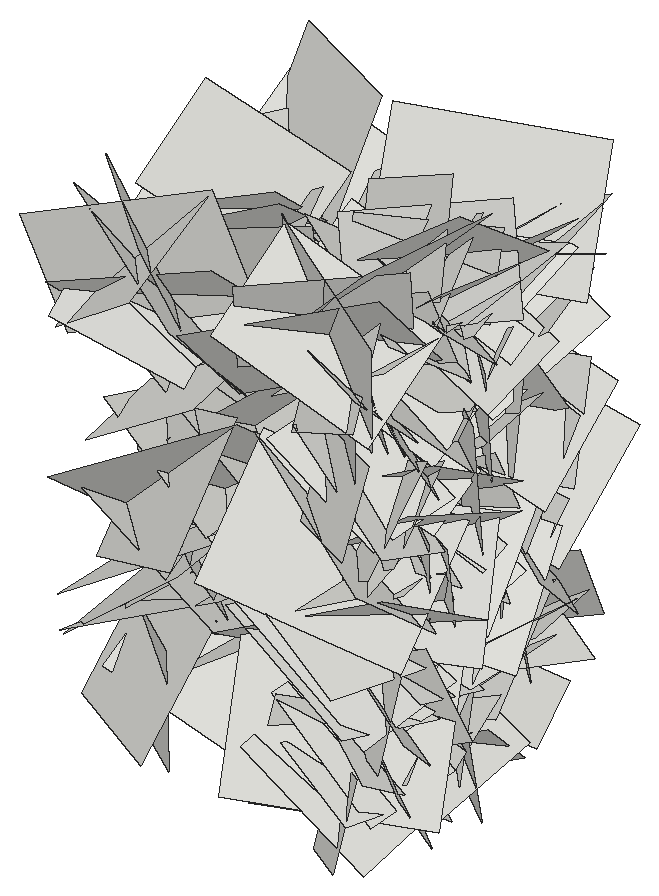
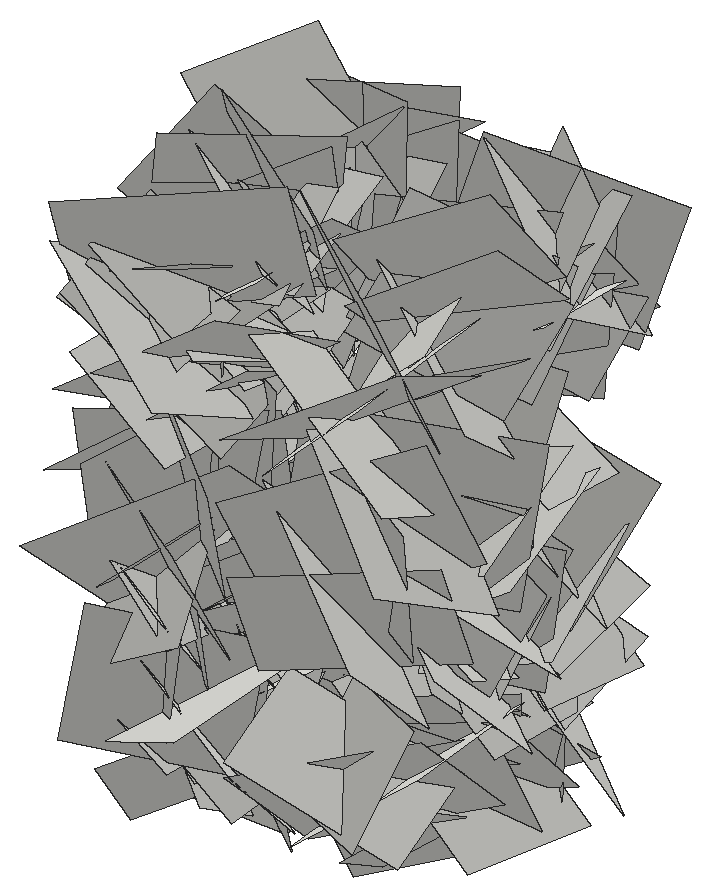
# SketchUp Ruby script. Lengths in inches.
U = 1.inch
M = Sketchup.active_model
def pt(a) = Geom::Point3d.new(a.map { |v| v * U })
def face(e, loops, mat)
  f = e.add_face(loops[0].map { |a| pt(a) })
  loops[1..].each { |l| e.add_face(l.map { |a| pt(a) }).erase! }
  f.material = f.back_material = mat if mat
  f
end
# faces: each face lists its corners as indices into pts; further lists are holes
def faces(e, pts, list, mat = nil) = list.each { |f| face(e, (f[0].is_a?(Array) ? f : [f]).map { |l| l.map { |i| pts[i] } }, mat) }
# xy, xz, yz: faces in a plane at the given z, y or x. An outline is a flat list of corners, or four numbers for a rectangle; further outlines are holes
def ring(l) = l.size == 4 ? [[l[0], l[1]], [l[2], l[1]], [l[2], l[3]], [l[0], l[3]]] : l.each_slice(2).to_a
def flat(e, list, mat, &to3) = list.each { |f| face(e, (f[0].is_a?(Array) ? f : [f]).map { |l| ring(l).map { |u, v| to3.(u, v) } }, mat) }
def xy(e, z, list, mat = nil) = flat(e, list, mat) { |x, y| [x, y, z] }
def xz(e, y, list, mat = nil) = flat(e, list, mat) { |x, z| [x, y, z] }
def yz(e, x, list, mat = nil) = flat(e, list, mat) { |y, z| [x, y, z] }
def lines(e, pts, list) = list.each { |a, b| e.add_line(pt(pts[a]), pt(pts[b])) }
# prism: a flat outline (further loops are holes) pulled along v
def prism(e, loops, v, mat = nil)
  f = face(e, loops, mat); d = Geom::Vector3d.new(v.map { |x| x * U })
  f.pushpull(f.normal.samedirection?(d) ? d.length : -d.length)
end
def box(e, o, s, mat = nil) = prism(e, [[o, [o[0] + s[0], o[1], o[2]], [o[0] + s[0], o[1] + s[1], o[2]], [o[0], o[1] + s[1], o[2]]]], [0, 0, s[2]], mat)
def at(x, y, z, deg = 0) = Geom::Transformation.translation(pt([x, y, z])) * Geom::Transformation.rotation(ORIGIN, Z_AXIS, deg.degrees)
def axes(o, x, y, z) = Geom::Transformation.new([*x, 0, *y, 0, *z, 0, *pt(o).to_a, 1])
def part(name) = M.definitions.add(name)
# library, detail: a bought-in or finely detailed component or shape, given as its bounding box
def library(name, o, s) = part(name).tap { |d| box(d.entities, o, s) }
def detail(e, o, s) = box(e.add_group.entities, o, s)
def put(e, d, t, mat = nil) = e.add_instance(d, t).tap { |i| i.material = mat if mat }
def group(e, t, mat = nil) = e.add_group.tap { |g| g.transformation = t; g.material = mat if mat }.entities
root = M.entities
c1 = part("Component\#6")
p = [[0.01,0,0],[0,3.24,4.54],[4.32,3.24,4.54],[4.33,0,0]]
faces(c1.entities,p,[[0,1,2,3]])
put(root,c1,axes([14.53,194.3,13.93],[-0.22437,-1.23478,-0.60854],[-0.19245,-0.58527,1.25072],[1.44644,-0.26941,0.07201]))
put(root,c1,axes([14.53,184.41,20.14],[-0.03821,-1.03167,-0.60174],[-0.15497,-0.59368,1.0266],[1.25647,-0.1046,0.10832]))
put(root,c1,axes([18.5,186.3,8.38],[-0.07617,0.47932,0.41871],[0.13681,0.42359,-0.46276],[-0.66062,0.03245,-0.14411]))
put(root,c1,axes([14.53,184.31,4.6],[0.1576,-0.1516,-1.0147],[-0.15202,-1.0183,0.13112],[1.07684,-0.12157,0.16702]))
put(root,c1,axes([14.53,179.32,18.3],[0.15069,0.54422,0.74866],[-0.00735,0.75804,-0.54972],[0.98107,-0.07791,-0.11911]))
put(root,c1,axes([18.5,188.8,6.44],[0.14743,-0.18272,-0.74199],[0.06403,-0.74919,0.19581],[-0.80747,-0.09277,-0.11994]))
put(root,c1,axes([14.53,185.52,6.2],[-0.2751,-0.65276,-1.16933],[-0.03559,-1.18754,0.67037],[1.41909,-0.15632,-0.20987]))
put(root,c1,axes([14.53,181.08,20.02],[-0.00536,1.00575,0.03656],[0.10796,0.03689,-1.00058],[1.06133,0.00133,0.10197]))
put(root,c1,axes([14.53,184.05,20.67],[0.10102,0.73684,0.6989],[-0.04073,0.70408,-0.73707],[1.07574,-0.04254,-0.09354]))
put(root,c1,axes([14.53,191.125,9.45],[-0.23474,-0.88576,-0.93612],[0.00151,-0.95001,0.89856],[1.36608,-0.15116,-0.16185]))
put(root,c1,axes([14.53,185.11,13.22],[0.08906,-0.95701,-0.12674],[0.0585,-0.12225,0.95969],[1.02162,0.09043,-0.0439]))
put(root,c1,axes([14.53,180.4,17.125],[-0.23878,-0.31981,1.17522],[0.15258,1.17979,0.34864],[1.28199,-0.19998,0.17739]))
put(root,c1,axes([14.53,187.48,17.59],[-0.04794,-0.78864,0.66349],[0.19289,0.64758,0.78214],[1.07529,-0.15133,-0.11072]))
put(root,c1,axes([14.53,187.26,9.21],[0.06299,-0.71122,-0.64775],[0.16214,-0.63375,0.70987],[1.00673,0.14657,-0.0738]))
put(root,c1,axes([18.5,191.11,1.26],[0.04561,-0.57908,-0.31344],[0.1156,-0.3035,0.57569],[-0.68833,-0.08935,0.07592]))
put(root,c1,axes([14.53,186.13,19.34],[0.13168,0.96657,0.23982],[0.01085,0.24043,-0.97432],[1.05558,-0.12304,-0.0199]))
put(root,c1,axes([14.53,188.68,19.83],[-0.08458,1.11358,0.50301],[-0.01593,0.50315,-1.11627],[1.29513,0.07891,0.01912]))
put(root,c1,axes([14.53,185.36,5.79],[0.02078,-1.22604,-0.15411],[-0.11589,-0.15525,1.22117],[1.3047,0.00574,0.11093]))
put(root,c1,axes([14.53,186.43,6.6],[-0.00451,1.27416,-0.10814],[-0.14001,-0.108,-1.26731],[1.34821,-0.00695,-0.13197]))
put(root,c1,axes([18.5,190.35,18.26],[0.16101,-0.65287,0.16772],[0.08445,0.18811,0.66008],[-0.7095,-0.12576,0.11663]))
put(root,c1,axes([14.53,187.9375,5.11],[0.04973,-1.23753,-0.07043],[-0.13139,-0.07481,1.23194],[1.30732,0.03956,0.12649]))
put(root,c1,axes([14.53,189.08,9.2],[-0.13088,0.55221,1.09741],[0.12619,1.10312,-0.54169],[1.29609,-0.05164,0.16356]))
put(root,c1,axes([14.53,182.44,13.63],[-0.1579,1.28482,-0.45217],[-0.02165,-0.45692,-1.2916],[1.44363,0.13368,-0.06883]))
put(root,c1,axes([14.53,182.53,23.48],[0.24403,0.37129,-0.99391],[-0.1038,-1.00526,-0.39821],[1.11985,-0.17408,0.17968]))
put(root,c1,axes([14.53,192.17,8.01],[0.17438,0.53527,-0.89237],[0.02164,-0.90494,-0.53904],[1.10282,-0.06688,0.15168]))
put(root,c1,axes([14.53,188.23,7.57],[0.0913,-1.12353,0.75234],[-0.27462,0.72618,1.11413],[1.40673,0.21468,0.16867]))
put(root,c1,axes([14.53,194.04,23.84],[-0.15699,-0.54259,-1.24113],[0.03696,-1.24964,0.54215],[1.43535,-0.02717,-0.14971]))
put(root,c1,axes([14.53,189.36,1.43],[-0.09807,-1.35815,-0.14277],[-0.05055,-0.1398,1.36078],[1.44669,-0.09695,0.03787]))
put(root,c1,axes([14.53,188.7,21.97],[0.14471,1.28216,-0.28655],[-0.25359,-0.25902,-1.27293],[1.36933,-0.18346,-0.20546]))
put(root,c1,axes([14.53,190.12,11.53],[-0.21117,-0.99907,-0.90649],[0.1512,-0.92678,0.99009],[1.42194,-0.04983,-0.2399]))
put(root,c1,axes([14.53,183.02,16.38],[-0.02893,-0.8566,0.75588],[0.26219,0.73373,0.84043],[1.18223,-0.18368,-0.16789]))
put(root,c1,axes([14.53,185.31,6.45],[-0.03902,-0.20515,1.15818],[0.22164,1.13915,0.20842],[1.22693,-0.21231,-0.00082]))
put(root,c1,axes([14.53,180.93,10.86],[-0.17521,1.15715,-0.62152],[0.20897,-0.59747,-1.1648],[1.37654,0.23798,0.09772]))
put(root,c1,axes([14.53,184.5,10.44],[0.20009,0.552,-0.98447],[-0.02572,-0.99592,-0.56307],[1.1961,-0.11375,0.15258]))
put(root,c1,axes([14.53,185.25,0.97],[0.15144,0.45294,1.0525],[0.02813,1.05906,-0.45936],[1.21425,-0.08102,-0.12063]))
put(root,c1,axes([14.53,182.38,2.76],[0.16715,0.82367,0.72398],[0.09449,0.71938,-0.83785],[1.15857,-0.1775,-0.03612]))
put(root,c1,axes([14.53,186.66,10.07],[-0.09303,-0.2424,1.37134],[-0.00293,1.37409,0.24271],[1.47615,-0.01254,0.08691]))
put(root,c1,axes([14.53,192.77,15.58],[0.03721,-0.16955,-1.17702],[0.1418,-1.1695,0.17246],[1.25252,0.13744,0.01545]))
put(root,c1,axes([14.53,185.87,11.99],[0.00632,-0.88407,-1.06115],[-0.10628,-1.05864,0.88141],[1.46017,-0.07323,0.06874]))
put(root,c1,axes([14.53,186.02,17.55],[0.12484,-0.91824,0.67786],[0.09261,0.68671,0.91505],[1.20627,0.04231,-0.14041]))
put(root,c1,axes([14.53,195.54,11.625],[0.04246,-1.00606,-0.92627],[-0.11693,-0.92602,1.00103],[1.44486,-0.04538,0.10823]))
put(root,c1,axes([14.53,183.88,15.08],[-0.0404,1.11797,-0.62329],[0.16276,-0.61507,-1.11262],[1.34698,0.10785,0.11575]))
put(root,c1,axes([14.53,184.23,21.55],[0.30098,0.54789,0.85036],[0.10123,0.86476,-0.58905],[1.06749,-0.23649,-0.1839]))
put(root,c1,axes([14.53,184,8.18],[-0.02134,-1.06466,0.81449],[0.04088,0.81378,1.06469],[1.42032,-0.03942,-0.01841]))
put(root,c1,axes([14.53,188.34,12.62],[0.20954,0.481,1.15591],[-0.07101,1.17261,-0.47649],[1.32521,-0.01322,-0.2083]))
put(root,c1,axes([14.53,186.39,13.5625],[0.22643,-0.80881,0.81079],[0.0736,0.83241,0.81208],[1.21171,0.10058,-0.20084]))
put(root,c1,axes([14.53,184.34,4.6],[0.11485,-1.15497,0.26483],[0.19184,0.27894,1.14248],[1.2413,0.06375,-0.20107]))
put(root,c1,axes([14.53,193.03,3.2],[0.23388,-1.096,0.27231],[0.13541,0.2999,1.10354],[1.1894,0.18138,-0.17918]))
put(root,c1,axes([14.53,189.55,17.94],[0.16397,-1.09761,-0.83604],[-0.11999,-0.84854,1.09307],[1.45761,0.05363,0.18403]))
put(root,c1,axes([14.53,187.39,3.1875],[0.10139,0.89849,0.89189],[0.1671,0.87902,-0.90243],[1.33152,-0.17873,0.04534]))
put(root,c1,axes([14.53,180.76,23.09],[0.06995,0.91309,-0.96842],[0.10566,-0.97028,-0.90805],[1.4069,0.02747,0.11634]))
put(root,c1,axes([14.53,183.54,2.14],[0.03864,0.84179,0.92004],[0.33491,0.88417,-0.82148],[1.27872,-0.257,0.18735]))
put(root,c1,axes([14.53,184.58,6.82],[0.16596,-1.29847,0.14138],[0.0614,0.14916,1.30572],[1.38315,0.14917,-0.07492]))
put(root,c1,axes([14.53,193.85,16.74],[0.30124,-1.14539,-0.57535],[-0.00001,-0.58933,1.17321],[1.35869,0.25394,0.12757]))
put(root,c1,axes([14.53,189.11,8.53],[0.25892,-1.11224,-0.53402],[0.14932,-0.51568,1.13849],[1.29927,0.28091,-0.02442]))
put(root,c1,axes([14.53,182.27,16.13],[0.23771,-0.47409,1.27281],[0.00404,1.29026,0.47991],[1.43973,0.07465,-0.2115]))
put(root,c1,axes([28.31,182.27,16.13],[-0.23771,-0.47409,1.27281],[-0.00404,1.29026,0.47991],[-1.43973,0.07465,-0.2115]))
put(root,c1,axes([28.31,189.11,8.53],[-0.25892,-1.11224,-0.53402],[-0.14932,-0.51568,1.13849],[-1.29927,0.28091,-0.02442]))
put(root,c1,axes([28.31,193.85,16.74],[-0.30124,-1.14539,-0.57535],[0.00001,-0.58933,1.17321],[-1.35869,0.25394,0.12757]))
put(root,c1,axes([28.31,184.58,6.82],[-0.16596,-1.29847,0.14138],[-0.0614,0.14916,1.30572],[-1.38315,0.14917,-0.07492]))
put(root,c1,axes([28.31,183.54,2.14],[-0.03864,0.84179,0.92004],[-0.33491,0.88417,-0.82148],[-1.27872,-0.257,0.18735]))
put(root,c1,axes([28.31,180.76,23.09],[-0.06995,0.91309,-0.96842],[-0.10566,-0.97028,-0.90805],[-1.4069,0.02747,0.11634]))
put(root,c1,axes([28.31,187.39,3.1875],[-0.10139,0.89849,0.89189],[-0.1671,0.87902,-0.90243],[-1.33152,-0.17873,0.04534]))
put(root,c1,axes([28.31,189.55,17.94],[-0.16397,-1.09761,-0.83604],[0.11999,-0.84854,1.09307],[-1.45761,0.05363,0.18403]))
put(root,c1,axes([28.31,193.03,3.2],[-0.23388,-1.096,0.27231],[-0.13541,0.2999,1.10354],[-1.1894,0.18138,-0.17918]))
put(root,c1,axes([28.31,184.34,4.6],[-0.11485,-1.15497,0.26483],[-0.19184,0.27894,1.14248],[-1.2413,0.06375,-0.20107]))
put(root,c1,axes([28.31,186.39,13.5625],[-0.22643,-0.80881,0.81079],[-0.0736,0.83241,0.81208],[-1.21171,0.10058,-0.20084]))
put(root,c1,axes([28.31,188.34,12.62],[-0.20954,0.481,1.15591],[0.07101,1.17261,-0.47649],[-1.32521,-0.01322,-0.2083]))
put(root,c1,axes([28.31,184,8.18],[0.02134,-1.06466,0.81449],[-0.04088,0.81378,1.06469],[-1.42032,-0.03942,-0.01841]))
put(root,c1,axes([28.31,184.23,21.55],[-0.30098,0.54789,0.85036],[-0.10123,0.86476,-0.58905],[-1.06749,-0.23649,-0.1839]))
put(root,c1,axes([28.31,183.88,15.08],[0.0404,1.11797,-0.62329],[-0.16276,-0.61507,-1.11262],[-1.34698,0.10785,0.11575]))
put(root,c1,axes([28.31,195.54,11.625],[-0.04246,-1.00606,-0.92627],[0.11693,-0.92602,1.00103],[-1.44486,-0.04538,0.10823]))
put(root,c1,axes([28.31,186.02,17.55],[-0.12484,-0.91824,0.67786],[-0.09261,0.68671,0.91505],[-1.20627,0.04231,-0.14041]))
put(root,c1,axes([28.31,185.87,11.99],[-0.00632,-0.88407,-1.06115],[0.10628,-1.05864,0.88141],[-1.46017,-0.07323,0.06874]))
put(root,c1,axes([28.31,192.77,15.58],[-0.03721,-0.16955,-1.17702],[-0.1418,-1.1695,0.17246],[-1.25252,0.13744,0.01545]))
put(root,c1,axes([28.31,186.66,10.07],[0.09303,-0.2424,1.37134],[0.00293,1.37409,0.24271],[-1.47615,-0.01254,0.08691]))
put(root,c1,axes([28.31,182.38,2.76],[-0.16715,0.82367,0.72398],[-0.09449,0.71938,-0.83785],[-1.15857,-0.1775,-0.03612]))
put(root,c1,axes([28.31,185.25,0.97],[-0.15144,0.45294,1.0525],[-0.02813,1.05906,-0.45936],[-1.21425,-0.08102,-0.12063]))
put(root,c1,axes([28.31,184.5,10.44],[-0.20009,0.552,-0.98447],[0.02572,-0.99592,-0.56307],[-1.1961,-0.11375,0.15258]))
put(root,c1,axes([28.31,180.93,10.86],[0.17521,1.15715,-0.62152],[-0.20897,-0.59747,-1.1648],[-1.37654,0.23798,0.09772]))
put(root,c1,axes([28.31,185.31,6.45],[0.03902,-0.20515,1.15818],[-0.22164,1.13915,0.20842],[-1.22693,-0.21231,-0.00082]))
put(root,c1,axes([28.31,183.02,16.38],[0.02893,-0.8566,0.75588],[-0.26219,0.73373,0.84043],[-1.18223,-0.18368,-0.16789]))
put(root,c1,axes([28.31,190.12,11.53],[0.21117,-0.99907,-0.90649],[-0.1512,-0.92678,0.99009],[-1.42194,-0.04983,-0.2399]))
put(root,c1,axes([28.31,188.7,21.97],[-0.14471,1.28216,-0.28655],[0.25359,-0.25902,-1.27293],[-1.36933,-0.18346,-0.20546]))
put(root,c1,axes([28.31,189.36,1.43],[0.09807,-1.35815,-0.14277],[0.05055,-0.1398,1.36078],[-1.44669,-0.09695,0.03787]))
put(root,c1,axes([28.31,194.04,23.84],[0.15699,-0.54259,-1.24113],[-0.03696,-1.24964,0.54215],[-1.43535,-0.02717,-0.14971]))
put(root,c1,axes([28.31,188.23,7.57],[-0.0913,-1.12353,0.75234],[0.27462,0.72618,1.11413],[-1.40673,0.21468,0.16867]))
put(root,c1,axes([28.31,192.17,8.01],[-0.17438,0.53527,-0.89237],[-0.02164,-0.90494,-0.53904],[-1.10282,-0.06688,0.15168]))
put(root,c1,axes([28.31,182.53,23.48],[-0.24403,0.37129,-0.99391],[0.1038,-1.00526,-0.39821],[-1.11985,-0.17408,0.17968]))
put(root,c1,axes([28.31,182.44,13.63],[0.1579,1.28482,-0.45217],[0.02165,-0.45692,-1.2916],[-1.44363,0.13368,-0.06883]))
put(root,c1,axes([28.31,189.08,9.2],[0.13088,0.55221,1.09741],[-0.12619,1.10312,-0.54169],[-1.29609,-0.05164,0.16356]))
put(root,c1,axes([28.31,187.9375,5.11],[-0.04973,-1.23753,-0.07043],[0.13139,-0.07481,1.23194],[-1.30732,0.03956,0.12649]))
put(root,c1,axes([24.34,190.35,18.26],[-0.16101,-0.65287,0.16772],[-0.08445,0.18811,0.66008],[0.7095,-0.12576,0.11663]))
put(root,c1,axes([28.31,186.43,6.6],[0.00451,1.27416,-0.10814],[0.14001,-0.108,-1.26731],[-1.34821,-0.00695,-0.13197]))
put(root,c1,axes([28.31,185.36,5.79],[-0.02078,-1.22604,-0.15411],[0.11589,-0.15525,1.22117],[-1.3047,0.00574,0.11093]))
put(root,c1,axes([28.31,188.68,19.83],[0.08458,1.11358,0.50301],[0.01593,0.50315,-1.11627],[-1.29513,0.07891,0.01912]))
put(root,c1,axes([28.31,186.13,19.34],[-0.13168,0.96657,0.23982],[-0.01085,0.24043,-0.97432],[-1.05558,-0.12304,-0.0199]))
put(root,c1,axes([24.34,191.11,1.26],[-0.04561,-0.57908,-0.31344],[-0.1156,-0.3035,0.57569],[0.68833,-0.08935,0.07592]))
put(root,c1,axes([28.31,187.26,9.21],[-0.06299,-0.71122,-0.64775],[-0.16214,-0.63375,0.70987],[-1.00673,0.14657,-0.0738]))
put(root,c1,axes([28.31,187.48,17.59],[0.04794,-0.78864,0.66349],[-0.19289,0.64758,0.78214],[-1.07529,-0.15133,-0.11072]))
put(root,c1,axes([28.31,180.4,17.125],[0.23878,-0.31981,1.17522],[-0.15258,1.17979,0.34864],[-1.28199,-0.19998,0.17739]))
put(root,c1,axes([28.31,185.11,13.22],[-0.08906,-0.95701,-0.12674],[-0.0585,-0.12225,0.95969],[-1.02162,0.09043,-0.0439]))
put(root,c1,axes([28.31,191.125,9.45],[0.23474,-0.88576,-0.93612],[-0.00151,-0.95001,0.89856],[-1.36608,-0.15116,-0.16185]))
put(root,c1,axes([28.31,184.05,20.67],[-0.10102,0.73684,0.6989],[0.04073,0.70408,-0.73707],[-1.07574,-0.04254,-0.09354]))
put(root,c1,axes([28.31,181.08,20.02],[0.00536,1.00575,0.03656],[-0.10796,0.03689,-1.00058],[-1.06133,0.00133,0.10197]))
put(root,c1,axes([28.31,185.52,6.2],[0.2751,-0.65276,-1.16933],[0.03559,-1.18754,0.67037],[-1.41909,-0.15632,-0.20987]))
put(root,c1,axes([24.34,188.8,6.44],[-0.14743,-0.18272,-0.74199],[-0.06403,-0.74919,0.19581],[0.80747,-0.09277,-0.11994]))
put(root,c1,axes([28.31,179.32,18.3],[-0.15069,0.54422,0.74866],[0.00735,0.75804,-0.54972],[-0.98107,-0.07791,-0.11911]))
put(root,c1,axes([28.31,184.31,4.6],[-0.1576,-0.1516,-1.0147],[0.15202,-1.0183,0.13112],[-1.07684,-0.12157,0.16702]))
put(root,c1,axes([24.34,186.3,8.38],[0.07617,0.47932,0.41871],[-0.13681,0.42359,-0.46276],[0.66062,0.03245,-0.14411]))
put(root,c1,axes([28.31,184.41,20.14],[0.03821,-1.03167,-0.60174],[0.15497,-0.59368,1.0266],[-1.25647,-0.1046,0.10832]))
put(root,c1,axes([28.31,194.3,13.93],[0.22437,-1.23478,-0.60854],[0.19245,-0.58527,1.25072],[-1.44644,-0.26941,0.07201]))
put(root,c1,axes([24.34,187.98,11.49],[-0.12716,0.81746,0.20835],[-0.15,0.18797,-0.81896],[0.88154,0.1499,-0.10929]))
put(root,c1,axes([24.34,186.0625,6.1],[-0.08854,0.52684,0.45627],[0.00383,0.45985,-0.53032],[0.73876,0.06076,0.05744]))
put(root,c1,axes([28.31,181.29,16.68],[-0.08133,-0.245,0.96212],[0.05676,0.96256,0.24939],[-1.05086,0.07095,-0.06099]))
put(root,c1,axes([28.31,184.19,13.53],[-0.08078,-0.49886,0.79857],[-0.01528,0.8017,0.49945],[-0.99796,0.02811,-0.07229]))
put(root,c1,axes([28.31,187.61,11.62],[0.28203,-0.58282,-1.12773],[-0.01249,-1.15332,0.59327],[-1.34554,-0.11146,-0.24188]))
put(root,c1,axes([24.34,183.1,18.89],[-0.1435,0.17311,-0.85276],[-0.14536,-0.85648,-0.1521],[0.91084,-0.10941,-0.15862]))
put(root,c1,axes([24.34,183.83,7.3125],[-0.02805,0.62389,-0.09529],[0.05665,-0.09282,-0.62253],[0.66659,0.03414,0.0489]))
put(root,c1,axes([28.31,184.51,1.15],[0.01173,-1.06899,-0.22188],[0.10644,-0.21996,1.06472],[-1.15237,-0.0312,0.09608]))
put(root,c1,axes([28.31,186.9375,3.03],[-0.11563,0.62873,-0.58509],[-0.05581,-0.59358,-0.62803],[-0.90867,-0.04354,0.11303]))
put(root,c1,axes([24.34,189.45,1.42],[0.1039,0.30381,0.53974],[-0.07033,0.54846,-0.29667],[0.65275,0.01074,-0.11787]))
put(root,c1,axes([24.34,184.54,3.47],[-0.05739,0.5962,-0.42459],[-0.0201,-0.42675,-0.59681],[0.77559,0.03305,-0.04688]))
put(root,c1,axes([28.31,185.64,19.96],[0.2349,1.07139,0.39402],[-0.08081,0.41437,-1.08385],[-1.20734,0.18072,0.1492]))
put(root,c1,axes([28.31,186.72,4.72],[0.08241,-0.91883,0.29273],[-0.13826,0.28096,0.91654],[-1.0128,-0.11312,-0.1013]))
put(root,c1,axes([28.31,190.33,17.67],[-0.17424,0.82504,0.17436],[0.04616,0.18571,-0.83769],[-0.89267,-0.15144,-0.07735]))
put(root,c1,axes([28.31,179.97,24.47],[0.23304,1.36821,0.06434],[0.25904,0.02493,-1.36533],[-1.42861,0.2277,-0.23708]))
put(root,c1,axes([24.34,184.43,15.42],[-0.12844,-0.04329,0.74472],[0.08874,0.74892,0.05716],[0.78574,-0.09166,0.11528]))
put(root,c1,axes([28.31,189.57,16.9],[-0.06471,0.53395,-0.71324],[-0.01751,-0.71546,-0.53421],[-0.94426,-0.02333,0.05878]))
put(root,c1,axes([28.31,191,16.96],[0.17643,-1.14926,-0.11809],[0.05518,-0.11173,1.16072],[-1.22339,-0.17078,0.03532]))
put(root,c1,axes([24.34,186.92,8.78],[-0.10246,-0.30095,0.75916],[-0.04625,0.76527,0.29782],[0.86439,0.00528,0.10592]))
put(root,c1,axes([28.31,180.14,11.99],[0.0212,0.75168,0.8023],[0.17372,0.79143,-0.74558],[-1.15236,0.13314,-0.09764]))
put(root,c1,axes([28.31,185.08,2.16],[-0.06404,-1.02262,-0.11109],[0.17979,-0.11966,1.00929],[-1.07543,0.04089,0.17535]))
put(root,c1,axes([28.31,187.17,12.95],[0.05814,-0.16279,1.09674],[0.14666,1.09051,0.15494],[-1.1661,0.12904,0.07417]))
put(root,c1,axes([28.31,187.85,22.99],[-0.09057,-0.06637,-0.91857],[0.07612,-0.92019,0.05981],[-0.97325,-0.06579,0.09016]))
put(root,c1,axes([24.34,183.375,2.21],[0.01982,-0.33114,-0.74136],[-0.16849,-0.7287,0.32148],[0.84401,-0.13769,0.08159]))
put(root,c1,axes([24.34,192.83,7.86],[0.1126,-0.65912,-0.17655],[-0.1088,-0.19208,0.65534],[0.71507,0.07456,0.12751]))
put(root,c1,axes([28.31,183.46,7.83],[0.1867,0.36795,-0.96583],[-0.13041,-0.96532,-0.39019],[-1.08777,0.17888,-0.11899]))
put(root,c1,axes([28.31,186.63,-0.64],[0.14781,-0.37723,1.01914],[0.01271,1.02797,0.37886],[-1.15185,-0.03706,0.13496]))
put(root,c1,axes([28.31,183.61,1.59],[-0.06331,-0.78644,0.46242],[0.03597,0.46118,0.7887],[-0.96639,0.06869,-0.00094]))
put(root,c1,axes([28.31,185.25,15.47],[-0.04372,0.77316,0.71524],[0.20224,0.70943,-0.75587],[-1.09798,0.09988,-0.16771]))
put(root,c1,axes([28.31,185.13,2.21],[-0.09174,0.69928,0.36],[-0.10121,0.35015,-0.7031],[-0.82753,-0.12035,0.04608]))
put(root,c1,axes([24.34,192.38,19.24],[0.04943,-0.7355,0.057],[-0.07325,0.05251,0.73407],[0.77853,0.05163,0.06545]))
put(root,c1,axes([28.31,181.6,11.88],[-0.05183,0.72565,0.67247],[0.15864,0.67097,-0.71314],[-1.03662,0.0664,-0.14276]))
put(root,c1,axes([24.34,185.26,12.26],[-0.159,0.84642,0.10737],[0.04855,0.11685,-0.85715],[0.9031,0.14274,0.06498]))
put(root,c1,axes([24.34,185.94,13.1875],[-0.12339,0.16979,-0.82402],[0.01755,-0.83125,-0.17361],[0.89164,0.03986,-0.11061]))
put(root,c1,axes([24.34,183.19,13.8],[-0.02762,0.65605,0.3231],[0.06014,0.32414,-0.6536],[0.77284,-0.00178,0.06241]))
put(root,c1,axes([28.31,184.53,11.29],[0.10396,-0.95246,0.37472],[0.04499,0.37989,0.95451],[-1.084,-0.07558,0.07555]))
put(root,c1,axes([28.31,192.08,20.31],[-0.05296,-0.67773,-0.30339],[-0.1724,-0.2867,0.66724],[-0.76797,0.11109,-0.12886]))
put(root,c1,axes([24.34,192.03,8.33],[-0.03388,0.22508,-0.86549],[-0.13142,-0.8588,-0.21876],[0.93879,-0.1121,-0.06186]))
put(root,c1,axes([24.34,185.14,8.49],[0.08576,-0.66072,-0.04627],[0.0456,-0.04128,0.66459],[0.70059,0.08356,-0.03759]))
put(root,c1,axes([24.34,183.28,17.73],[-0.09647,-0.26045,0.74001],[0.11879,0.73302,0.27177],[0.82305,-0.13632,0.04751]))
put(root,c1,axes([24.34,193.37,9.31],[-0.05697,-0.46717,-0.61186],[0.09106,-0.61316,0.46062],[0.81091,0.03603,-0.09471]))
put(root,c1,axes([24.34,191.46,9.82],[-0.08538,-0.06629,-0.92063],[-0.09555,-0.91915,0.07407],[0.97372,-0.09601,-0.07345]))
put(root,c1,axes([24.34,191.35,2.27],[-0.06694,-0.86655,-0.10749],[-0.04783,-0.10439,0.86806],[0.92435,-0.06816,0.03713]))
put(root,c1,axes([24.34,190.84,12.42],[0.00848,-0.77925,-0.15089],[-0.03038,-0.15108,0.77873],[0.8408,0.0024,0.02966]))
put(root,c1,axes([24.34,182.98,9.92],[0.09782,-0.62966,-0.10425],[0.08997,-0.09229,0.63256],[0.67052,0.10424,-0.06967]))
put(root,c1,axes([24.34,180.19,4.07],[0.08532,0.68038,-0.07405],[0.04058,-0.07892,-0.68351],[0.72433,-0.07573,0.04702]))
put(root,c1,axes([24.34,183.91,5.17],[-0.1157,0.58195,-0.7538],[-0.08085,-0.76164,-0.57696],[1.0062,0.00571,-0.13304]))
put(root,c1,axes([24.34,182.875,15.8],[-0.04284,-0.30855,-0.78276],[-0.017,-0.78324,0.30957],[0.8917,-0.02976,-0.0317]))
put(root,c1,axes([28.31,184.33,2.33],[0.23495,-0.78095,0.69461],[-0.033,0.70481,0.80235],[-1.10738,-0.18669,0.12346]))
put(root,c1,axes([28.31,189.86,21.06],[0.09411,0.75469,-0.30292],[-0.23058,-0.27158,-0.74036],[-0.83059,0.16091,0.17121]))
put(root,c1,axes([28.31,189.65,5.54],[-0.06955,0.77959,0.08211],[-0.00823,0.08175,-0.78235],[-0.8309,-0.06607,0.00087]))
put(root,c1,axes([28.31,192.04,5.47],[0.24252,-0.79203,0.72828],[0.0092,0.7459,0.80846],[-1.14049,-0.1624,0.16139]))
put(root,c1,axes([28.31,184.16,21.8125],[0.07155,0.99261,-0.10082],[0.11355,-0.10768,-0.9884],[-1.05147,0.05592,-0.1136]))
put(root,c1,axes([24.34,184.68,7.1],[-0.07537,-0.21143,-0.85755],[-0.01444,-0.85996,0.21315],[0.93612,-0.03029,-0.06575]))
put(root,c1,axes([24.34,187.95,18.35],[-0.24952,-0.85217,0.60628],[-0.01294,0.62364,0.87183],[1.1085,-0.18454,0.14665]))
put(root,c1,axes([28.31,188.38,23.95],[0.14683,-0.05211,-1.06804],[0.1506,-1.06652,0.07046],[-1.12342,-0.14978,-0.13015]))
